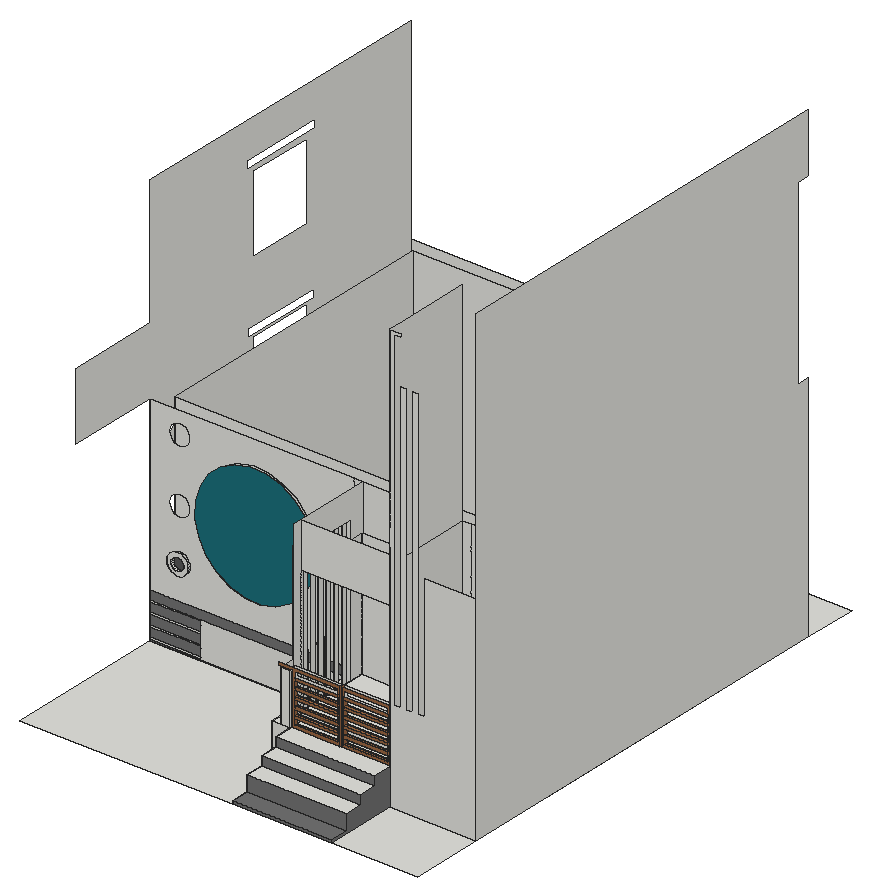
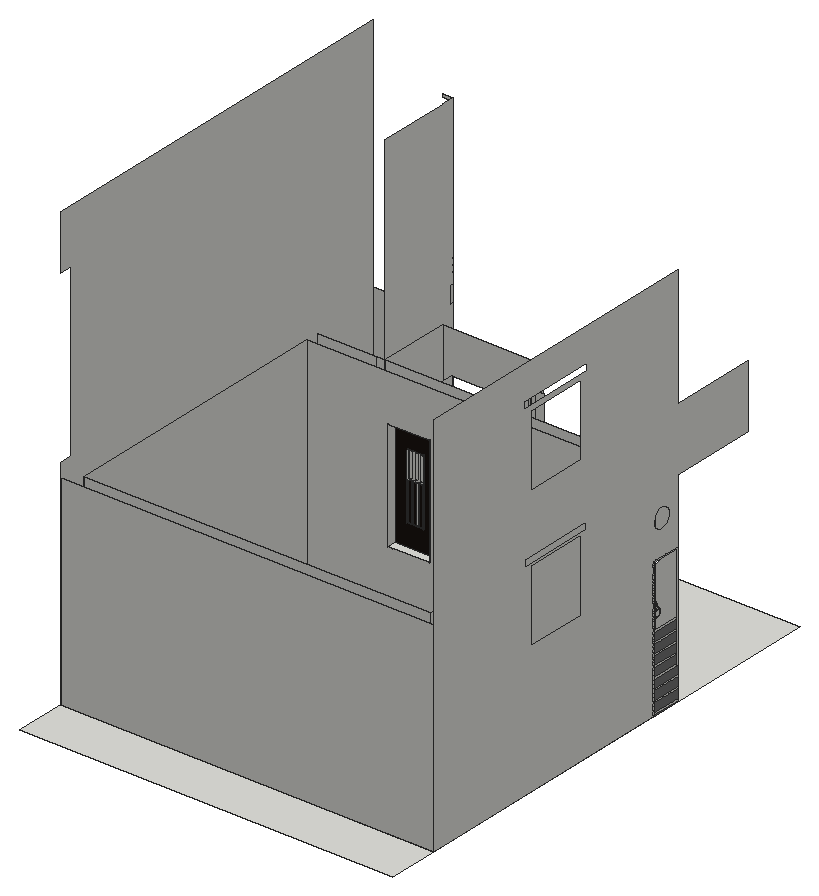
# SketchUp Ruby script. Lengths in inches.
U = 1.inch
M = Sketchup.active_model
def pt(a) = Geom::Point3d.new(a.map { |v| v * U })
def face(e, loops, mat)
  f = e.add_face(loops[0].map { |a| pt(a) })
  loops[1..].each { |l| e.add_face(l.map { |a| pt(a) }).erase! }
  f.material = f.back_material = mat if mat
  f
end
# faces: each face lists its corners as indices into pts; further lists are holes
def faces(e, pts, list, mat = nil) = list.each { |f| face(e, (f[0].is_a?(Array) ? f : [f]).map { |l| l.map { |i| pts[i] } }, mat) }
# xy, xz, yz: faces in a plane at the given z, y or x. An outline is a flat list of corners, or four numbers for a rectangle; further outlines are holes
def ring(l) = l.size == 4 ? [[l[0], l[1]], [l[2], l[1]], [l[2], l[3]], [l[0], l[3]]] : l.each_slice(2).to_a
def flat(e, list, mat, &to3) = list.each { |f| face(e, (f[0].is_a?(Array) ? f : [f]).map { |l| ring(l).map { |u, v| to3.(u, v) } }, mat) }
def xy(e, z, list, mat = nil) = flat(e, list, mat) { |x, y| [x, y, z] }
def xz(e, y, list, mat = nil) = flat(e, list, mat) { |x, z| [x, y, z] }
def yz(e, x, list, mat = nil) = flat(e, list, mat) { |y, z| [x, y, z] }
def lines(e, pts, list) = list.each { |a, b| e.add_line(pt(pts[a]), pt(pts[b])) }
# prism: a flat outline (further loops are holes) pulled along v
def prism(e, loops, v, mat = nil)
  f = face(e, loops, mat); d = Geom::Vector3d.new(v.map { |x| x * U })
  f.pushpull(f.normal.samedirection?(d) ? d.length : -d.length)
end
def box(e, o, s, mat = nil) = prism(e, [[o, [o[0] + s[0], o[1], o[2]], [o[0] + s[0], o[1] + s[1], o[2]], [o[0], o[1] + s[1], o[2]]]], [0, 0, s[2]], mat)
def at(x, y, z, deg = 0) = Geom::Transformation.translation(pt([x, y, z])) * Geom::Transformation.rotation(ORIGIN, Z_AXIS, deg.degrees)
def axes(o, x, y, z) = Geom::Transformation.new([*x, 0, *y, 0, *z, 0, *pt(o).to_a, 1])
def part(name) = M.definitions.add(name)
# library, detail: a bought-in or finely detailed component or shape, given as its bounding box
def library(name, o, s) = part(name).tap { |d| box(d.entities, o, s) }
def detail(e, o, s) = box(e.add_group.entities, o, s)
def put(e, d, t, mat = nil) = e.add_instance(d, t).tap { |i| i.material = mat if mat }
def group(e, t, mat = nil) = e.add_group.tap { |g| g.transformation = t; g.material = mat if mat }.entities
root = M.entities
M.materials.add("I06_Sapphire_Night").color = [28, 110, 122]
M.materials.add("M05_Graphite_Haze").color = [114, 114, 114]
M.materials.add("M06_Steel_Smoke").color = [86, 86, 86]
M.materials.add("Wood_Floor_12_1K").color = [28, 22, 19]
M.materials.add("Wood_Veneer_15_1K").color = [153, 102, 66]
xy(root,0,[[18.64,0,159.64,0,159.64,48,147.64,48,147.64,108,18.64,108],[225.64,0,282.64,48],[[18.64,108,282.64,324],[27.64,117,273.64,315]],[27.64,117,273.64,315],[18.64,324,282.64,360]])
xy(root,1.95,[[159.64,0,225.64,12]],"M05_Graphite_Haze")
xy(root,12,[[159.64,12,225.64,24]])
xy(root,17.36,[[158.35,59.83,158.94,62.61],[158.35,66.32,158.94,69.11],[158.35,72.81,158.94,75.6],[158.35,79.31,158.94,82.09],[158.35,85.8,158.94,88.58],
  [158.35,92.29,158.94,95.07]])
xy(root,18,[[159.64,24,225.64,36]])
xy(root,21.38,[[151.68,61.7,152.875,63.02],[151.68,69.7,152.875,71.02],[151.68,77.69,152.875,79.01],[151.68,85.6875,152.875,87.01],[151.68,93.68,152.875,95]])
xy(root,24,[[159.64,36,225.64,36,225.64,48.875,193.14,48.875,193.14,50.875,192.14,50.875,192.14,48.875,159.64,48.875],[147.64,48,153.64,48,153.64,58,159.64,58,159.64,98,153.64,98,153.64,108,147.64,108],[159.64,48.875,192.14,50.875],[193.14,48.875,225.64,50.875],[159.64,50.875,225.64,56.88],
  [159.64,56.88,225.64,108]])
xy(root,24.31,[[151.68,101.68,152.875,103]])
xy(root,26,[[161.64,48.875,190.64,50.875],[194.64,48.875,223.64,50.875]],"Wood_Veneer_15_1K")
xy(root,29.67,[[161.64,48.875,190.64,50.875],[194.64,48.875,223.64,50.875]])
xy(root,30,[[159.64,56.88,219.64,107]])
xy(root,30,[[183.64,107,219.64,108]],"Wood_Veneer_15_1K")
xy(root,31.67,[[161.64,48.875,190.64,50.875],[194.64,48.875,223.64,50.875]],"Wood_Veneer_15_1K")
xy(root,33,[[186.64,110.5,216.64,117]])
xy(root,33,[[186.64,107,216.64,110.5]],"Wood_Veneer_15_1K")
xy(root,35.33,[[161.64,48.875,190.64,50.875],[194.64,48.875,223.64,50.875]])
xy(root,37.33,[[161.64,48.875,190.64,50.875],[194.64,48.875,223.64,50.875]],"Wood_Veneer_15_1K")
xy(root,41,[[161.64,48.875,190.64,50.875],[194.64,48.875,223.64,50.875]])
xy(root,43,[[161.64,48.875,190.64,50.875],[194.64,48.875,223.64,50.875]],"Wood_Veneer_15_1K")
xy(root,46.67,[[161.64,48.875,190.64,50.875],[194.64,48.875,223.64,50.875]])
xy(root,47.74,[[196.19,109.5,208.59,110.5]])
xy(root,48.67,[[161.64,48.875,190.64,50.875],[194.64,48.875,223.64,50.875]],"Wood_Veneer_15_1K")
xy(root,48.74,[[197.19,109.5,199.99,110.5],[200.99,109.5,203.79,110.5],[204.79,109.5,207.59,110.5]])
xy(root,52.33,[[161.64,48.875,190.64,50.875],[194.64,48.875,223.64,50.875]])
xz(root,0,[[159.64,0,225.64,1.95]],"M05_Graphite_Haze")
xz(root,12,[[159.64,1.95,225.64,12]],"M05_Graphite_Haze")
xz(root,24,[[159.64,12,225.64,18]],"M05_Graphite_Haze")
xz(root,36,[[159.64,18,225.64,24]],"M05_Graphite_Haze")
xz(root,48,[[147.64,0,159.64,24],[225.64,0,282.64,0,282.64,144,248.68,144,248.68,62.04,244.33,62.04,244.33,252.41,240.8,252.41,240.8,61.91,236.45,61.91,236.45,252.41,232.92,252.41,232.92,61.78,228.57,61.78,228.57,281.97,232.92,281.97,232.92,284.15,225.72,284,225.72,274,225.64,274,225.64,154,225.72,154,225.72,144,225.64,144],[153.64,24,159.64,58.02]])
xz(root,48.875,[[159.64,24,192.14,24,192.14,60,151.11,60,151.11,58,190.64,58,190.64,26,161.64,26,161.64,58,159.64,58],[[193.14,24,225.64,60],[194.64,26,223.64,58]],[161.64,29.67,190.64,31.67],[194.64,29.67,223.64,31.67],[161.64,35.33,190.64,37.33],
  [194.64,35.33,223.64,37.33],[161.64,41,190.64,43],[194.64,41,223.64,43],[161.64,46.67,190.64,48.67],[194.64,46.67,223.64,48.67],
  [161.64,52.33,190.64,54.33],[194.64,52.33,223.64,54.33]],"Wood_Veneer_15_1K")
xz(root,50.875,[[[159.64,24,192.14,60],[161.64,43,190.64,46.67],[161.64,26,190.64,29.67],[161.64,54.33,190.64,58],[161.64,48.67,190.64,52.33],[161.64,37.33,190.64,41],[161.64,31.67,190.64,35.33]],[[193.14,24,225.64,60],[194.64,43,223.64,46.67],[194.64,26,223.64,29.67],[194.64,54.33,223.64,58],[194.64,48.67,223.64,52.33],[194.64,37.33,223.64,41],[194.64,31.67,223.64,35.33]]])
xz(root,56.88,[[159.64,24,225.64,24,225.64,144,159.64,144,159.64,114,219.64,114,219.64,30,159.64,30]])
xz(root,58,[[153.64,24,153.64,126,159.64,126,159.64,99.18,157.14,99.18,157.14,93.95,159.64,93.95,159.64,24]])
xz(root,59.83,[[158.35,17.36,158.94,126]])
xz(root,61.7,[[151.68,21.38,152.875,58]],"Wood_Veneer_15_1K")
xz(root,62.61,[[158.35,17.36,158.94,126]])
xz(root,63.02,[[151.68,21.38,152.875,58]],"Wood_Veneer_15_1K")
xz(root,66.32,[[158.35,17.36,158.94,126]])
xz(root,69.11,[[158.35,17.36,158.94,126]])
xz(root,69.7,[[151.68,21.38,152.875,58]],"Wood_Veneer_15_1K")
xz(root,71.02,[[151.68,21.38,152.875,58]])
xz(root,72.81,[[158.35,17.36,158.94,126]])
xz(root,75.6,[[158.35,17.36,158.94,126]])
xz(root,77.69,[[151.68,21.38,152.875,58]],"Wood_Veneer_15_1K")
xz(root,79.01,[[151.68,21.38,152.875,58]])
xz(root,79.31,[[158.35,17.36,158.94,126]])
xz(root,82.09,[[158.35,17.36,158.94,126]])
xz(root,85.6875,[[151.68,21.38,152.875,58]],"Wood_Veneer_15_1K")
xz(root,85.8,[[158.35,17.36,158.94,126]])
xz(root,87.01,[[151.68,21.38,152.875,58]])
xz(root,88.58,[[158.35,17.36,158.94,126]])
xz(root,92.29,[[158.35,17.36,158.94,126]])
xz(root,93.68,[[151.68,21.38,152.875,58]],"Wood_Veneer_15_1K")
xz(root,95,[[151.68,21.38,152.875,58]])
xz(root,95.07,[[158.35,17.36,158.94,126]])
xz(root,98,[[153.64,24,159.64,24,159.64,93.95,157.14,93.95,157.14,99.18,159.64,99.18,159.64,126,153.64,126]])
xz(root,101.68,[[151.68,24.31,152.875,58]],"Wood_Veneer_15_1K")
xz(root,103,[[151.68,24.31,152.875,58]])
xz(root,106,[[[38.08,46.23,39.89,46.41,41.6,47.06,43.08,48.12,44.24,49.53,44.99,51.19,45.29,52.99,45.11,54.81,44.46,56.52,43.4,58,41.99,59.15,40.33,59.91,38.53,60.2,36.71,60.02,35,59.38,33.52,58.32,32.37,56.9,31.61,55.24,31.32,53.44,31.5,51.625,32.14,49.92,33.21,48.4375,34.62,47.28,36.28,46.53],[38.3,48.97,37.2,49.12,36.18,49.54,35.3,50.22,34.625,51.1,34.2,52.12,34.06,53.22,34.2,54.32,34.625,55.34,35.3,56.22,36.18,56.89,37.2,57.32,38.3,57.46,39.4,57.32,40.43,56.89,41.3,56.22,41.98,55.34,42.4,54.32,42.55,53.22,42.4,52.12,41.98,51.1,41.3,50.22,40.43,49.54,39.4,49.12]]])
xz(root,106,[[93.35,48.6,103.54,50.83,112.8,55.62,120.51,62.64,126.14,71.42,129.3,81.35,129.79,91.77,127.5625,101.95,122.78,111.21,115.75,118.92,106.98,124.55,97.04,127.72,86.63,128.2,76.44,125.98,67.18,121.19,59.47,114.17,53.84,105.39,50.68,95.46,50.19,85.04,52.42,74.86,57.2,65.59,64.22,57.88,73,52.26,82.9375,49.09]],"I06_Sapphire_Night")
xz(root,107,[[159.64,30,183.64,114]])
xz(root,107,[[[183.64,30,219.64,114],[186.64,33,216.64,111]]],"Wood_Veneer_15_1K")
xz(root,108,[[51.95,0,147.64,24],[147.64,0,159.64,0,159.64,144,153.64,144,153.64,24,147.64,24],[159.64,0,225.64,24],[225.64,0,231.64,144],[231.64,0,273.64,144],
  [18.64,1,51.95,2],[18.64,8.45,51.95,9.45],[18.64,15.89,51.95,16.89],[18.64,23.34,51.95,24],[[159.64,24,225.64,144],[183.64,30,219.64,114]],
  [[18.64,30,153.64,144],[93.35,48.6,82.9375,49.09,73,52.26,64.22,57.88,57.2,65.59,52.42,74.86,50.19,85.04,50.68,95.46,53.84,105.39,59.47,114.17,67.18,121.19,76.44,125.98,86.63,128.2,97.04,127.72,106.98,124.55,115.75,118.92,122.78,111.21,127.5625,101.95,129.79,91.77,129.3,81.35,126.14,71.42,120.51,62.64,112.8,55.62,103.54,50.83],[38.08,122.25,36.28,122.54,34.62,123.29,33.21,124.45,32.14,125.93,31.5,127.64,31.32,129.45,31.61,131.25,32.37,132.92,33.52,134.33,35,135.39,36.71,136.04,38.53,136.22,40.33,135.92,41.99,135.17,43.4,134.01,44.46,132.53,45.11,130.82,45.29,129.01,44.99,127.21,44.24,125.54,43.08,124.13,41.6,123.07,39.89,122.43],[38.08,80.04,36.28,80.34,34.62,81.09,33.21,82.25,32.14,83.73,31.5,85.4375,31.32,87.25,31.61,89.05,32.37,90.71,33.52,92.125,35,93.1875,36.71,93.83,38.53,94.01,40.33,93.72,41.99,92.96,43.4,91.81,44.46,90.33,45.11,88.62,45.29,86.8,44.99,85,44.24,83.34,43.08,81.93,41.6,80.87,39.89,80.22],[38.08,46.23,36.28,46.53,34.62,47.28,33.21,48.4375,32.14,49.92,31.5,51.625,31.32,53.44,31.61,55.24,32.37,56.9,33.52,58.32,35,59.38,36.71,60.02,38.53,60.2,40.33,59.91,41.99,59.15,43.4,58,44.46,56.52,45.11,54.81,45.29,52.99,44.99,51.19,44.24,49.53,43.08,48.12,41.6,47.06,39.89,46.41]]])
xz(root,108,[[18.64,0,51.95,1],[18.64,2,51.95,8.45],[18.64,9.45,51.95,15.89],[18.64,16.89,51.95,23.34],[18.64,24,153.64,30]],"M05_Graphite_Haze")
xz(root,108,[[38.3,48.97,39.4,49.12,40.43,49.54,41.3,50.22,41.98,51.1,42.4,52.12,42.55,53.22,42.4,54.32,41.98,55.34,41.3,56.22,40.43,56.89,39.4,57.32,38.3,57.46,37.2,57.32,36.18,56.89,35.3,56.22,34.625,55.34,34.2,54.32,34.06,53.22,34.2,52.12,34.625,51.1,35.3,50.22,36.18,49.54,37.2,49.12]],"M06_Steel_Smoke")
xz(root,109.5,[[[196.19,47.74,208.59,95.34],[204.79,48.74,204.79,75.66,207.59,75.66,207.59,76.43,204.79,76.43,204.79,94.34,207.59,94.34,207.59,48.74],[200.99,48.74,203.79,75.66],[197.19,48.74,199.99,75.66],[200.99,76.43,203.79,94.34],[197.19,76.43,199.99,94.34]]])
xz(root,110.5,[[[186.64,33,216.64,111],[196.19,47.74,208.59,95.34]],[197.19,48.74,199.99,75.66],[200.99,48.74,203.79,75.66],[204.79,48.74,207.59,75.66]],"Wood_Floor_12_1K")
xz(root,117,[[[27.64,0,273.64,144],[186.64,33,216.64,111]]])
xz(root,315,[[27.64,0,273.64,144]])
xz(root,324,[[18.64,0,282.64,144]])
yz(root,18.64,[[[129.87,0,129.87,98.35,108,98.35,108,144,46,144,46,189,108,189,108,274,324,274,324,0],[193.5,92.42,237.59,143.3],[193.5,190.875,237.59,241.76],[187.98,244.92,244.27,250.47],[189.1,144.51,243.39,149.79],[122.03,116,123.83,116.3,125.5,117.05,126.91,118.2,127.97,119.6875,128.62,121.39,128.8,123.21,128.5,125.01,127.75,126.67,126.59,128.08,125.11,129.14,123.4,129.79,121.59,129.97,119.79,129.67,118.125,128.92,116.71,127.76,115.65,126.28,115.01,124.58,114.83,122.76,115.12,120.96,115.875,119.3,117.03,117.89,118.51,116.82,120.22,116.18]],[128.87,0,128.87,97.35,109,97.35,109,23.34,108,23.34,108,98.35,129.87,98.35,129.87,0],[108,1,128.87,2],[108,8.45,128.87,9.45],[108,15.89,128.87,16.89],
  [109,23.34,128.87,24.34],[109,30.78,128.87,31.78],[109,38.23,128.87,39.23],[109,45.67,128.87,46.67],[109,53.12,128.87,54.12]])
yz(root,18.64,[[108,0,128.87,1],[108,2,128.87,8.45],[108,9.45,128.87,15.89],[108,16.89,128.87,23.34],[109,24.34,128.87,30.78],
  [109,31.78,128.87,38.23],[109,39.23,128.87,45.67],[109,46.67,128.87,53.12]],"M05_Graphite_Haze")
yz(root,27.64,[[117,0,315,144]])
yz(root,147.64,[[48,0,108,24]])
yz(root,151.68,[[61.7,21.38,63.02,58],[69.7,21.38,71.02,58],[77.69,21.38,79.01,58],[85.6875,21.38,87.01,58],[93.68,21.38,95,58],
  [101.68,24.31,103,58]],"Wood_Veneer_15_1K")
yz(root,152.875,[[61.7,21.38,63.02,58],[69.7,21.38,71.02,58],[77.69,21.38,79.01,58],[85.6875,21.38,87.01,58],[93.68,21.38,95,58],
  [101.68,24.31,103,58]])
yz(root,153.64,[[48,24,48,58.02,50.875,58.02,50.875,58,58,58,58,24],[98,24,108,58]])
yz(root,158.35,[[59.83,17.36,62.61,126],[66.32,17.36,69.11,126],[72.81,17.36,75.6,126],[79.31,17.36,82.09,126],[85.8,17.36,88.58,126],
  [92.29,17.36,95.07,126]])
yz(root,158.94,[[59.83,17.36,62.61,126],[66.32,17.36,69.11,126],[72.81,17.36,75.6,126],[79.31,17.36,82.09,126],[85.8,17.36,88.58,126],
  [92.29,17.36,95.07,126]])
yz(root,159.64,[[48,24,48.875,58.02],[48.875,24,50.875,58],[50.875,24,56.88,144],[56.88,24,58,30],[98,24,98,30,107,30,107,114,98,114,98,126,58,126,58,114,56.88,114,56.88,144,108,144,108,24],
  [58,24,98,30],[56.88,30,58,114],[98,30,107,114]])
yz(root,159.64,[[0,0,12,1.95],[12,0,12,12,24,12,24,18,36,18,36,24,48,24,48,0]],"M05_Graphite_Haze")
yz(root,161.64,[[48.875,26,50.875,29.67],[48.875,31.67,50.875,35.33],[48.875,37.33,50.875,41],[48.875,43,50.875,46.67],[48.875,48.67,50.875,52.33]],"Wood_Veneer_15_1K")
yz(root,183.64,[[107,30,108,114]],"Wood_Veneer_15_1K")
yz(root,186.64,[[110.5,33,117,111]])
yz(root,186.64,[[107,33,110.5,111]],"Wood_Veneer_15_1K")
yz(root,190.64,[[48.875,26,50.875,29.67],[48.875,31.67,50.875,35.33],[48.875,37.33,50.875,41],[48.875,43,50.875,46.67],[48.875,48.67,50.875,52.33]],"Wood_Veneer_15_1K")
yz(root,192.14,[[48.875,24,50.875,60]],"Wood_Veneer_15_1K")
yz(root,193.14,[[48.875,24,50.875,60]],"Wood_Veneer_15_1K")
yz(root,194.64,[[48.875,26,50.875,29.67],[48.875,31.67,50.875,35.33],[48.875,37.33,50.875,41],[48.875,43,50.875,46.67],[48.875,48.67,50.875,52.33]],"Wood_Veneer_15_1K")
yz(root,196.19,[[109.5,47.74,110.5,95.34]])
yz(root,197.19,[[109.5,48.74,110.5,75.66]])
yz(root,199.99,[[109.5,48.74,110.5,75.66]])
yz(root,200.99,[[109.5,48.74,110.5,75.66]])
yz(root,203.79,[[109.5,48.74,110.5,75.66]])
yz(root,204.79,[[109.5,48.74,110.5,75.66]])
yz(root,207.59,[[109.5,48.74,110.5,75.66]])
yz(root,208.59,[[109.5,47.74,110.5,48.74],[109.5,48.74,110.5,94.34]])
yz(root,216.64,[[110.5,33,117,111]])
yz(root,216.64,[[107,33,110.5,111]],"Wood_Veneer_15_1K")
yz(root,219.64,[[56.88,30,107,114]])
yz(root,219.64,[[107,30,108,114]],"Wood_Veneer_15_1K")
yz(root,223.64,[[48.875,26,50.875,29.67],[48.875,31.67,50.875,35.33],[48.875,37.33,50.875,41],[48.875,43,50.875,46.67],[48.875,48.67,50.875,52.33]])
yz(root,225.64,[[48,24,48,154,51,154,51,166,48,166,48,169.1,49.04,169.1,49.04,170.1,48,170.1,48,173.43,49.04,173.43,49.04,174.42,48,174.42,48,177.75,49.04,177.75,49.04,178.74,48,178.74,48,182.08,49.04,182.08,49.04,183.07,48,183.07,48,186.4,49.04,186.4,49.04,187.39,48,187.39,48,284.16,57,284.16,57,284,108,284,108,144,56.88,144,56.88,24,50.875,24,50.875,60,48.875,60,48.875,24],[48.875,24,50.875,60],[56.88,24,108,144]])
yz(root,225.64,[[0,0,48,0,48,24,36,24,36,18,24,18,24,12,12,12,12,1.95,0,1.95]],"M05_Graphite_Haze")
yz(root,273.64,[[117,0,315,144]])
yz(root,282.64,[[48,0,324,0,324,154,315,154,315,274,324,274,324,313.32,48,313.32]])
p = [[36.28,108,46.53],[38.08,108,46.23],[38.08,106,46.23],[36.28,106,46.53],[39.89,108,46.41],[39.89,106,46.41],
  [41.6,108,47.06],[41.6,106,47.06],[34.62,108,47.28],[34.62,106,47.28],[43.08,108,48.12],[43.08,106,48.12],
  [33.21,108,48.4375],[33.21,106,48.4375],[44.24,108,49.53],[44.24,106,49.53],[32.14,108,49.92],[32.14,106,49.92],
  [82.9375,108,49.09],[93.35,108,48.6],[93.35,106,48.6],[82.9375,106,49.09],[103.54,108,50.83],[103.54,106,50.83],
  [38.3,108,48.97],[37.2,108,49.12],[37.2,106,49.12],[38.3,106,48.97],[39.4,108,49.12],[39.4,106,49.12],
  [36.18,108,49.54],[36.18,106,49.54],[40.43,108,49.54],[40.43,106,49.54],[73,108,52.26],[73,106,52.26],
  [35.3,108,50.22],[35.3,106,50.22],[41.3,108,50.22],[41.3,106,50.22],[44.99,108,51.19],[44.99,106,51.19],
  [31.5,108,51.625],[31.5,106,51.625],[34.625,108,51.1],[34.625,106,51.1],[41.98,108,51.1],[41.98,106,51.1],
  [112.8,108,55.62],[112.8,106,55.62],[34.2,108,52.12],[34.2,106,52.12],[42.4,108,52.12],[42.4,106,52.12],
  [45.29,108,52.99],[45.29,106,52.99],[31.32,108,53.44],[31.32,106,53.44],[34.06,108,53.22],[34.06,106,53.22],
  [42.55,108,53.22],[42.55,106,53.22],[64.22,108,57.88],[64.22,106,57.88],[45.11,108,54.81],[45.11,106,54.81],
  [34.2,108,54.32],[34.2,106,54.32],[42.4,108,54.32],[42.4,106,54.32],[31.61,108,55.24],[31.61,106,55.24]]
faces(root,p,[[0,1,2,3],[1,4,5,2],[4,6,7,5],[8,0,3,9],[6,10,11,7],[12,8,9,13],[10,14,15,11],[16,12,13,17],
  [18,19,20,21],[19,22,23,20],[24,25,26,27],[28,24,27,29],[25,30,31,26],[32,28,29,33],[34,18,21,35],[30,36,37,31],
  [38,32,33,39],[14,40,41,15],[42,16,17,43],[36,44,45,37],[46,38,39,47],[22,48,49,23],[44,50,51,45],[52,46,47,53],
  [40,54,55,41],[56,42,43,57],[50,58,59,51],[60,52,53,61],[62,34,35,63],[54,64,65,55],[58,66,67,59],[68,60,61,69],
  [70,56,57,71]])
